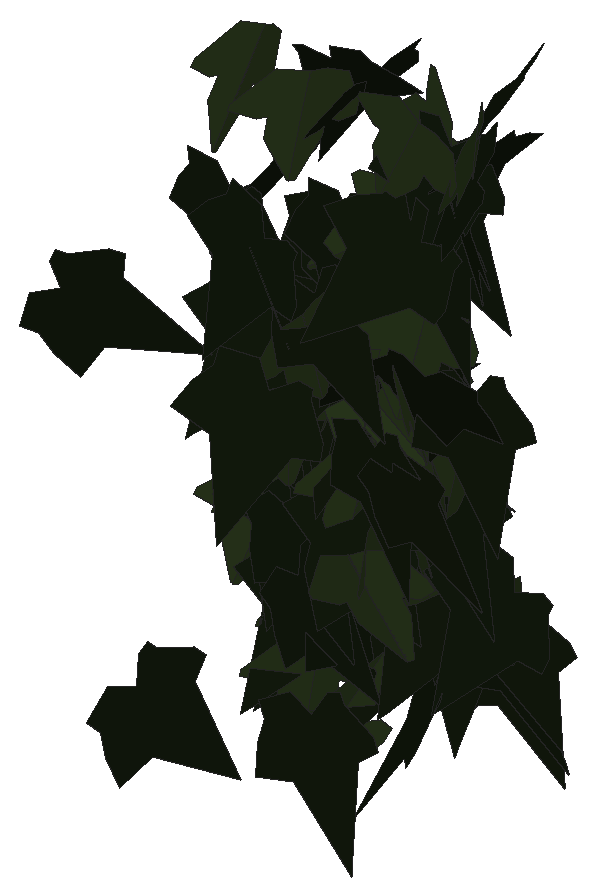
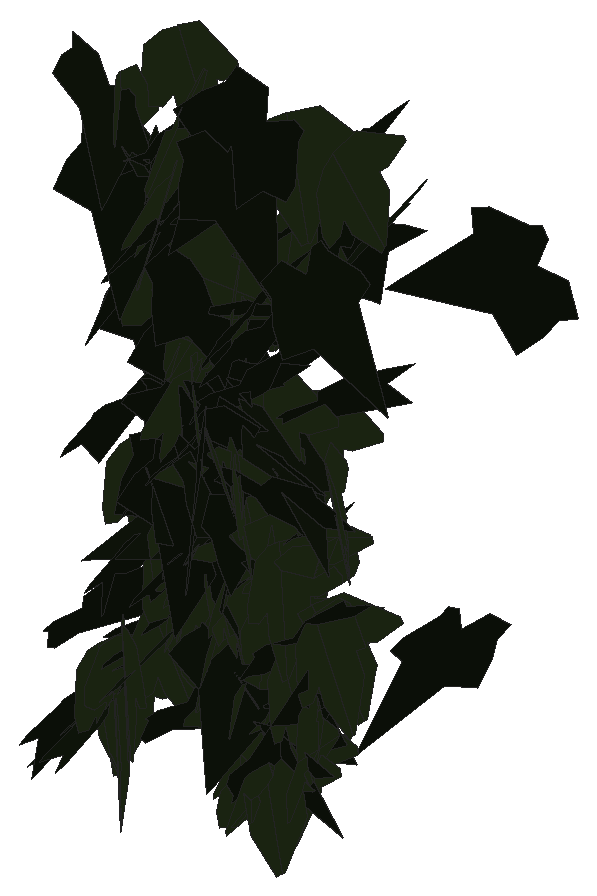
# SketchUp Ruby script. Lengths in inches.
U = 1.inch
M = Sketchup.active_model
def pt(a) = Geom::Point3d.new(a.map { |v| v * U })
def face(e, loops, mat)
  f = e.add_face(loops[0].map { |a| pt(a) })
  loops[1..].each { |l| e.add_face(l.map { |a| pt(a) }).erase! }
  f.material = f.back_material = mat if mat
  f
end
# faces: each face lists its corners as indices into pts; further lists are holes
def faces(e, pts, list, mat = nil) = list.each { |f| face(e, (f[0].is_a?(Array) ? f : [f]).map { |l| l.map { |i| pts[i] } }, mat) }
# xy, xz, yz: faces in a plane at the given z, y or x. An outline is a flat list of corners, or four numbers for a rectangle; further outlines are holes
def ring(l) = l.size == 4 ? [[l[0], l[1]], [l[2], l[1]], [l[2], l[3]], [l[0], l[3]]] : l.each_slice(2).to_a
def flat(e, list, mat, &to3) = list.each { |f| face(e, (f[0].is_a?(Array) ? f : [f]).map { |l| ring(l).map { |u, v| to3.(u, v) } }, mat) }
def xy(e, z, list, mat = nil) = flat(e, list, mat) { |x, y| [x, y, z] }
def xz(e, y, list, mat = nil) = flat(e, list, mat) { |x, z| [x, y, z] }
def yz(e, x, list, mat = nil) = flat(e, list, mat) { |y, z| [x, y, z] }
def lines(e, pts, list) = list.each { |a, b| e.add_line(pt(pts[a]), pt(pts[b])) }
# prism: a flat outline (further loops are holes) pulled along v
def prism(e, loops, v, mat = nil)
  f = face(e, loops, mat); d = Geom::Vector3d.new(v.map { |x| x * U })
  f.pushpull(f.normal.samedirection?(d) ? d.length : -d.length)
end
def box(e, o, s, mat = nil) = prism(e, [[o, [o[0] + s[0], o[1], o[2]], [o[0] + s[0], o[1] + s[1], o[2]], [o[0], o[1] + s[1], o[2]]]], [0, 0, s[2]], mat)
def at(x, y, z, deg = 0) = Geom::Transformation.translation(pt([x, y, z])) * Geom::Transformation.rotation(ORIGIN, Z_AXIS, deg.degrees)
def axes(o, x, y, z) = Geom::Transformation.new([*x, 0, *y, 0, *z, 0, *pt(o).to_a, 1])
def part(name) = M.definitions.add(name)
# library, detail: a bought-in or finely detailed component or shape, given as its bounding box
def library(name, o, s) = part(name).tap { |d| box(d.entities, o, s) }
def detail(e, o, s) = box(e.add_group.entities, o, s)
def put(e, d, t, mat = nil) = e.add_instance(d, t).tap { |i| i.material = mat if mat }
def group(e, t, mat = nil) = e.add_group.tap { |g| g.transformation = t; g.material = mat if mat }.entities
root = M.entities
M.materials.add("efeu1").color = [18, 25, 13]
M.materials.add("efeu2").color = [43, 57, 29]
c1 = part("ivyleaf_10")
p = [[0,0.5,-0.03],[-0.0625,2.02,-0.43],[-0.19,2.01,-0.46],[-0.54,1.05,-0.29],[-0.52,0.625,-0.18],[-0.83,0.76,-0.28],
  [-1.16,0.64,-0.33],[-1.15,0.33,-0.24],[-0.77,-0.39,0.02],[-0.3,-0.51,0.16],[0.04,-0.48,0.23],[-0.02,2.01,-0.4375],
  [-0.06,2.01,-0.43],[0.04,-0.49,0.23],[0.67,-0.49,0.14],[1.38,0.36,-0.2],[1.375,0.51,-0.24],[0.81,0.65,-0.19],
  [0.62,0.59,-0.15],[0.6,1.09,-0.28],[0.5,1.23,-0.31]]
faces(c1.entities,p,[[0,1,2,3,4,5,6,7,8,9,10],[11,12,0,13,14,15,16,17,18,19,20]],"efeu2")
c2 = part("ivyleaf_9")
p = [[1.54,2.16,1.25],[1.36,2.04,1.19],[-0.21,0.99,0.68],[-0.71,1.11,0.82],[-0.85,0.86,0.67],[-0.8,0.17,0.21],
  [-0.9,-0.01,0.1],[-0.67,-0.16,-0.02],[-0.08,-0.08,-0.05],[-0.03,-0.6,-0.4],[0.65,-0.88,-0.66],[0.83,-0.6,-0.49],
  [1.29,-0.42,-0.43],[1.8125,-0.07,-0.26],[1.21,0.44,0.15]]
faces(c2.entities,p,[[0,1,2,3,4,5,6,7,8,9,10,11,12,13,14]],"efeu1")
put(root,c1,axes([19.44,222.39,243.55],[-0.01108,-0.49032,0.09727],[0.0069,-0.09743,-0.49037],[0.49983,-0.00952,0.00893]))
put(root,c2,axes([19.07,219.82,246.48],[0.1213,0.02445,-0.48445],[0.28717,0.39883,0.09203],[0.39092,-0.30056,0.08272]))
put(root,c1,axes([19.42,222.27,245.14],[0.30029,-0.39808,0.03688],[0.05716,-0.0029,-0.49671],[0.39568,0.30253,0.04376]))
put(root,c1,axes([19.6,222.22,243.52],[-0.27833,-0.36558,0.19719],[-0.0556,-0.20243,-0.45379],[0.41163,-0.27454,0.07203]))
put(root,c1,axes([19.41,222.78,242.53],[-0.01774,0.17283,-0.46884],[0.04454,-0.46673,-0.17373],[-0.4977,-0.04793,0.00117]))
put(root,c1,axes([19.51,221.99,248.25],[-0.02394,-0.44074,0.23489],[0.06215,-0.23596,-0.43642],[0.49555,0.0083,0.06608]))
put(root,c2,axes([19.79,222.18,247.12],[-0.2297,0.38883,-0.2146],[0.05063,-0.2171,-0.44755],[-0.44122,-0.22733,0.06036]))
put(root,c1,axes([19.65,222.62,243.16],[0.06523,-0.49538,0.01862],[-0.00038,-0.01883,-0.49965],[0.49573,0.06517,-0.00284]))
put(root,c2,axes([19.8,222.8,242.26],[-0.17445,-0.39074,0.25862],[0.10442,0.23661,0.42792],[-0.4568,0.20331,-0.00095]))
put(root,c1,axes([19.82,222.78,242.22],[-0.21532,-0.44772,0.05641],[-0.00416,-0.06054,-0.4963],[0.45124,-0.21419,0.02235]))
put(root,c2,axes([19.69,222.5,243.53],[-0.13385,-0.48058,0.03356],[-0.00506,-0.03343,-0.49886],[0.48172,-0.13388,0.00408]))
put(root,c1,axes([19.87,222.46,244.17],[-0.04913,-0.4925,-0.07091],[0.00897,0.07037,-0.49494],[0.4975,-0.04991,0.00192]))
put(root,c1,axes([19.83,222.76,242.27],[-0.0214,0.43846,-0.23937],[-0.0254,-0.24024,-0.43777],[-0.4989,-0.00657,0.03255]))
put(root,c2,axes([20.02,222.71,242.46],[-0.48575,-0.09263,-0.07392],[0.07164,0.01896,-0.49448],[0.09441,-0.49098,-0.00515]))
put(root,c1,axes([19.79,222.09,244.13],[0.15451,0.47129,0.06333],[0.02774,0.05754,-0.4959],[-0.47472,0.15676,-0.00836]))
put(root,c2,axes([19.79,220.01,242.45],[0.12581,-0.20795,-0.43696],[-0.10901,0.4277,-0.23493],[0.47148,0.15437,0.06228]))
put(root,c1,axes([20.26,222.06,244.17],[0.15449,0.07499,0.46958],[-0.43453,-0.17831,0.17143],[0.19317,-0.46107,0.01008]))
put(root,c1,axes([20,222.74,242.77],[0.04949,-0.47561,-0.14609],[0.00177,0.14698,-0.47791],[0.49754,0.04679,0.01623]))
put(root,c2,axes([20.02,222.51,242.54],[-0.29711,-0.387,0.10934],[-0.07569,-0.0797,-0.48777],[0.39496,-0.3064,-0.01122]))
put(root,c2,axes([19.98,221.75,245.61],[-0.27657,-0.37553,0.18025],[-0.03623,-0.19385,-0.45947],[0.41497,-0.2672,0.08002]))
put(root,c1,axes([19.91,222.74,242.55],[-0.02184,0.47886,-0.14219],[-0.00742,-0.14262,-0.47917],[-0.49947,-0.01882,0.01334]))
put(root,c2,axes([20.31,221.9,245.15],[-0.17916,0.44858,0.12916],[-0.09313,0.10122,-0.48071],[-0.45742,-0.1963,0.04729]))
put(root,c2,axes([20.17,222.72,243.14],[0.04789,0.44383,0.22522],[-0.01794,0.22765,-0.44481],[-0.49738,0.03452,0.03773]))
put(root,c2,axes([19.82,221.3125,247.09],[0.05028,-0.46421,0.17883],[0.06656,-0.17185,-0.4648],[0.49299,0.07054,0.04452]))
put(root,c2,axes([20.06,222.5,244.98],[-0.37971,-0.25936,-0.19636],[0.1894,0.06913,-0.45755],[0.26448,-0.42185,0.04575]))
put(root,c1,axes([20.14,222.54,242.63],[-0.07016,-0.46182,-0.17832],[0.02959,0.17586,-0.46711],[0.49417,-0.07609,0.00265]))
put(root,c1,axes([20.23,222.07,242.07],[-0.29212,-0.40137,0.05969],[-0.02394,-0.05638,-0.49623],[0.40508,-0.29278,0.01372]))
put(root,c1,axes([20.09,222.56,242.85],[0.239,0.43915,0.00562],[-0.01394,0.01398,-0.49961],[-0.43896,0.23865,0.01892]))
put(root,c1,axes([20.28,222.78,243.11],[0.11009,-0.48542,0.04737],[0.00036,-0.04848,-0.49764],[0.48773,0.10961,-0.01032]))
put(root,c1,axes([20.33,222.53,243.49],[-0.24429,-0.43621,0.0064],[0.00558,-0.01046,-0.49986],[0.43622,-0.24415,0.00998]))
put(root,c1,axes([20.26,222.62,244.34],[0.29357,0.36079,-0.18344],[-0.11088,-0.14625,-0.4651],[-0.38926,0.31375,-0.00587]))
put(root,c1,axes([20.35,221.75,248.21],[-0.28011,-0.4076,0.07346],[-0.01306,-0.07995,-0.49339],[0.41396,-0.27833,0.03414]))
put(root,c1,axes([20.32,222.48,244.96],[0.18695,-0.45958,-0.06195],[0.00746,0.06976,-0.49505],[0.46368,0.18417,0.03294]))
put(root,c1,axes([20.33,222.66,243.72],[0.0864,-0.36412,-0.33159],[0.03489,0.34033,-0.36463],[0.49124,0.03987,0.08422]))
put(root,c2,axes([20.41,222.58,244.78],[-0.27135,0.21259,-0.36218],[0.24815,-0.26671,-0.34247],[-0.33881,-0.36561,0.03923]))
put(root,c1,axes([20.41,221.39,245.09],[-0.23966,-0.4372,-0.03767],[0.01803,0.03308,-0.49858],[0.43845,-0.24033,-0.00009]))
put(root,c1,axes([20.31,222.57,244.125],[-0.32616,-0.29253,-0.24092],[0.18513,0.15436,-0.43806],[0.33067,-0.37496,0.00762]))
put(root,c1,axes([20.67,222.54,244.81],[-0.34121,-0.12798,0.34234],[-0.29268,-0.1848,-0.36081],[0.21889,-0.44662,0.0512]))
put(root,c2,axes([20.26,222.43,243.96],[-0.03911,-0.4848,0.11593],[0.01186,-0.11716,-0.48594],[0.49833,-0.03526,0.02066]))
put(root,c1,axes([20.53,221.96,245.49],[-0.40967,-0.27833,0.06855],[-0.05406,-0.0424,-0.49526],[0.28151,-0.4132,0.00465]))
put(root,c2,axes([20.24,222.33,246.53],[0.09876,-0.48312,-0.08273],[-0.02283,0.07976,-0.49307],[0.48962,0.10116,-0.0063]))
put(root,c1,axes([20.45,222.65,243.97],[0.15813,-0.46926,0.06925],[0.01817,-0.06695,-0.49516],[0.47399,0.15911,-0.00412]))
put(root,c2,axes([20.41,222.28,243.5625],[-0.17795,-0.42442,0.19545],[-0.03274,-0.1973,-0.45826],[0.46611,-0.1759,0.04243]))
put(root,c2,axes([20.65,222.28,248.15],[-0.13614,0.4645,-0.12533],[0.01024,-0.12742,-0.48338],[-0.481,-0.13418,0.02518]))
put(root,c2,axes([20.72,222.42,244.83],[-0.29607,0.39524,-0.07831],[0.01755,-0.08444,-0.49251],[-0.40254,-0.29438,0.03612]))
put(root,c2,axes([20.45,222.34,245.87],[-0.16839,-0.46104,0.09532],[-0.00206,-0.10051,-0.48979],[0.47079,-0.16535,0.03195]))
put(root,c1,axes([20.53,222.7,242.94],[0.47155,-0.15182,-0.06775],[-0.06398,0.02235,-0.49539],[0.15345,0.47587,0.00165]))
put(root,c1,axes([20.58,221.81,243.1875],[-0.01597,-0.49709,-0.05147],[0.00979,0.05118,-0.49728],[0.49965,-0.01689,0.00809]))
put(root,c2,axes([20.38,221.53,243.8125],[0.18912,-0.43981,-0.14423],[-0.02541,0.1457,-0.47763],[0.46216,0.18799,0.03275]))
put(root,c2,axes([20.56,222.25,245.15],[-0.37621,-0.24187,-0.22352],[0.25262,0.00578,-0.43145],[0.21129,-0.43757,0.11786]))
put(root,c2,axes([20.49,222.02,248.4375],[0.47303,0.15077,-0.05925],[-0.06593,0.01214,-0.49549],[-0.14797,0.47657,0.03136]))
put(root,c2,axes([20.47,222.23,246.58],[0.03775,-0.47721,0.14437],[-0.00067,-0.14483,-0.47856],[0.49857,0.03594,-0.01158]))
put(root,c2,axes([20.73,222.54,244.79],[0.12815,0.48264,0.02521],[-0.00525,0.02747,-0.49922],[-0.48327,0.12768,0.01211]))
put(root,c1,axes([20.53,222,244.99],[-0.40635,-0.15797,-0.24479],[0.23483,0.07106,-0.43567],[0.17243,-0.46904,0.01644]))
put(root,c1,axes([20.65,222.48,245.18],[0.31296,-0.38967,0.01466],[0.00471,-0.01502,-0.49975],[0.38991,0.31295,-0.00573]))
put(root,c1,axes([20.59,222.34,245.07],[0.33798,-0.36769,-0.0239],[0.08857,0.11255,-0.47905],[0.35767,0.31958,0.14122]))
put(root,c2,axes([20.83,222.5625,245.08],[0.21202,0.33327,-0.30656],[-0.21063,-0.22707,-0.39253],[-0.40085,0.29559,0.04411]))
put(root,c2,axes([20.79,222.33,245.73],[-0.35685,-0.32402,0.13293],[-0.06809,-0.12197,-0.48009],[0.34354,-0.36075,0.04292]))
put(root,c1,axes([20.67,222.31,243.91],[-0.19108,-0.42513,-0.18098],[0.12484,0.14106,-0.46316],[0.44487,-0.22218,0.05224]))
put(root,c2,axes([20.85,222.4,245.19],[0.14781,-0.07938,-0.47101],[-0.43443,0.18261,-0.16711],[0.19855,0.45864,-0.01499]))
put(root,c1,axes([20.65,222.61,244.23],[-0.09798,0.48155,-0.09224],[0.02822,-0.08837,-0.49132],[-0.48949,-0.10148,-0.00987]))
put(root,c2,axes([20.49,220.87,246.72],[0.08299,-0.19606,0.45241],[0.16082,-0.42292,-0.21278],[0.4661,0.18083,-0.00714]))
put(root,c2,axes([20.98,222.48,244.66],[-0.2317,0.43701,-0.0731],[0.04618,-0.05822,-0.49445],[-0.44066,-0.23587,-0.01338]))
put(root,c2,axes([20.64,221.93,242.79],[-0.08495,-0.2996,0.39118],[0.0647,-0.4003,-0.29254],[0.48846,0.00091,0.10678]))
put(root,c1,axes([20.83,222.01,244.32],[-0.13573,-0.46731,0.1149],[0.02859,-0.12701,-0.48275],[0.48038,-0.12448,0.0612]))
put(root,c2,axes([20.75,220.58,247.26],[-0.0847,-0.41999,0.25775],[-0.05127,-0.25259,-0.42845],[0.4901,-0.09901,-0.00027]))
put(root,c1,axes([21.08,222.36,246.82],[-0.11343,-0.17,0.45632],[-0.25151,-0.38076,-0.20437],[0.41698,-0.27591,0.00086]))
put(root,c2,axes([20.8,222.66,242.55],[-0.19954,-0.44635,0.10465],[-0.01141,-0.10926,-0.48778],[0.45832,-0.19705,0.03341]))
put(root,c1,axes([20.76,222.56,244.73],[0.2168,0.38763,0.22966],[0.00996,0.25068,-0.43251],[-0.45044,0.19211,0.10097]))
put(root,c2,axes([20.9,222.22,246.38],[-0.35759,-0.3463,0.04694],[0.0389,-0.10618,-0.48704],[0.34729,-0.34468,0.10288]))
put(root,c2,axes([20.72,221.23,243.38],[0.25285,-0.33028,-0.27746],[-0.12544,0.25141,-0.41359],[0.41271,0.27876,0.04428]))
put(root,c2,axes([20.68,222.79,244.24],[0.11433,-0.48223,-0.06621],[0.00902,0.0701,-0.49498],[0.48667,0.11199,0.02473]))
put(root,c2,axes([20.94,222.05,243.6875],[-0.28575,-0.38621,0.13852],[-0.07885,-0.11396,-0.48041],[0.40265,-0.2964,0.00423]))
put(root,c1,axes([20.8125,221.46,241.59],[-0.08473,-0.42835,0.24359],[0.04011,0.24035,0.4366],[-0.49113,0.09352,-0.00637]))
put(root,c1,axes([21.01,222.42,243.86],[-0.2823,-0.36867,0.18544],[-0.06568,-0.18168,-0.46117],[0.40742,-0.28474,0.05415]))
put(root,c2,axes([21.0625,222.31,246.89],[-0.17276,0.3963,-0.2512],[0.11427,-0.22409,-0.43212],[-0.45508,-0.20672,-0.01314]))
put(root,c2,axes([21.09,222.41,245.55],[-0.47771,-0.13089,-0.06829],[0.06547,0.0195,-0.49531],[0.13232,-0.48217,-0.00149]))
put(root,c1,axes([20.99,222.3,245.66],[0.21326,-0.44513,-0.07985],[0.01109,0.0934,-0.49107],[0.4521,0.20768,0.04971]))
put(root,c2,axes([20.82,222.54,245.51],[-0.22081,-0.22187,-0.38989],[0.279,0.27238,-0.313],[0.35129,-0.35579,0.00351]))
put(root,c2,axes([20.6875,222.59,244.59],[0.431,-0.24877,0.04846],[0.10378,0.086,-0.48149],[0.23123,0.42511,0.12577]))
put(root,c1,axes([21.03,222.46,245.65],[-0.09934,0.48517,0.06889],[-0.07529,0.05435,-0.4913],[-0.48421,-0.10798,0.06226]))
put(root,c1,axes([21,221.83,246.83],[-0.35166,0.32937,-0.13361],[0.04985,-0.14039,-0.47729],[-0.35193,-0.34901,0.0659]))
put(root,c1,axes([21.04,222.04,246.42],[-0.46367,0.08486,-0.16677],[0.1659,-0.01963,-0.47126],[-0.08654,-0.49235,-0.00995]))
put(root,c1,axes([21.15,220.72,246.43],[-0.09944,-0.45925,-0.1709],[0.05084,0.16377,-0.46967],[0.48737,-0.11078,0.01412]))
put(root,c1,axes([21.13,222.32,243.65],[-0.32561,0.3674,-0.09484],[0.05905,-0.07438,-0.4909],[-0.37482,-0.33088,0.00505]))
put(root,c1,axes([20.82,221.87,245.23],[0.22743,0.04939,0.44253],[0.43576,0.07751,-0.23261],[-0.09158,0.49148,-0.00779]))
put(root,c2,axes([21.01,222.59,245.01],[0.10976,-0.48774,-0.00756],[-0.00753,0.00605,-0.49991],[0.48775,0.10986,-0.00601]))
put(root,c1,axes([21.49,222.14,244.6],[-0.24431,0.16957,0.40194],[-0.36625,0.17055,-0.29457],[-0.237,-0.43836,0.04088]))
put(root,c2,axes([21.33,221.62,245.74],[0.13573,0.48035,-0.02898],[-0.00889,-0.0276,-0.49916],[-0.48114,0.13602,0.00105]))
put(root,c2,axes([21.23,220.0625,246.03],[-0.22668,-0.44566,0.00276],[-0.00241,-0.00186,-0.49999],[0.44566,-0.22669,-0.0013]))
put(root,c1,axes([21.33,221.56,244.08],[0.20483,-0.41152,-0.19671],[0.02003,0.22354,-0.4468],[0.45568,0.17515,0.10806]))
put(root,c2,axes([21.09,222.71,243.1],[0.32576,-0.32061,-0.20271],[-0.04363,0.23376,-0.43983],[0.37679,0.30425,0.12432]))
put(root,c2,axes([21.11,220.96,246.61],[0.18673,-0.43657,-0.15665],[0.00245,0.1698,-0.47028],[0.46382,0.17486,0.06555]))
put(root,c1,axes([21.36,222.99,242.31],[0.23296,-0.41817,-0.14443],[-0.0003,0.16308,-0.47266],[0.44242,0.2203,0.07573]))
put(root,c1,axes([21.41,222.3125,242.9375],[-0.0176,-0.48078,0.13615],[-0.00201,-0.13617,-0.4811],[0.49969,-0.01748,0.00286]))
put(root,c1,axes([21.37,222.86,242.96],[0.34498,-0.3501,-0.09175],[0.01418,0.13973,-0.47987],[0.36165,0.32848,0.10634]))
put(root,c1,axes([21.41,222.3,247.75],[-0.153,0.34519,0.32777],[0.13808,-0.2973,0.37755],[0.45555,0.20604,-0.00435]))
put(root,c1,axes([21.45,222.29,247.48],[-0.15441,0.47462,0.02996],[-0.0112,0.02786,-0.4991],[-0.47543,-0.1548,0.00203]))
put(root,c1,axes([21.44,221.22,243.73],[-0.46008,-0.10652,-0.16426],[0.16125,0.03172,-0.47222],[0.11102,-0.48749,0.00517]))
put(root,c1,axes([21.5625,222.61,242.66],[-0.12105,-0.46542,-0.13686],[0.02198,0.13565,-0.48074],[0.48463,-0.12241,-0.01238]))
put(root,c2,axes([21.52,222.37,243.06],[-0.21199,-0.42707,0.15057],[-0.02538,-0.15478,-0.47476],[0.45212,-0.20894,0.04395]))
put(root,c1,axes([21.62,222.88,242.68],[-0.02173,-0.49923,0.0173],[0.00001,-0.01732,-0.4997],[0.49953,-0.02171,0.00076]))
put(root,c1,axes([21.59,221.64,245.76],[-0.22429,0.44196,0.0661],[-0.04003,0.05379,-0.49548],[-0.44507,-0.22756,0.01125]))
put(root,c2,axes([21.45,222.33,247.14],[0.21478,-0.35952,-0.27316],[-0.11961,0.24638,-0.41832],[0.43539,0.24504,0.01984]))
put(root,c2,axes([21.43,222.53,244.03],[0.1413,-0.46343,-0.12356],[-0.03482,0.11856,-0.48449],[0.47835,0.14552,0.00123]))
put(root,c1,axes([21.68,222.31,244.59],[-0.08001,-0.49283,0.02678],[-0.00335,-0.02659,-0.49928],[0.49355,-0.08007,0.00096]))
put(root,c1,axes([21.91,221.4,248.42],[-0.42469,-0.01551,0.26343],[-0.26044,-0.05574,-0.42316],[0.04249,-0.49664,0.03927]))
put(root,c2,axes([21.48,220.44,242.52],[0.09365,-0.47916,-0.10787],[0.00146,0.11009,-0.48773],[0.49115,0.09104,0.02202]))
put(root,c1,axes([21.82,221.62,246.25],[-0.36543,-0.31934,0.12036],[-0.06234,-0.11091,-0.48354],[0.33552,-0.36841,0.04124]))
put(root,c2,axes([21.55,222.52,242.84],[0.01317,-0.49584,0.06302],[-0.00321,-0.06312,-0.49599],[0.49982,0.01266,-0.00484]))
put(root,c2,axes([21.84,222.24,247.63],[0.03306,0.4977,0.03471],[0.00024,0.03477,-0.49879],[-0.49891,0.033,0.00206]))
put(root,c2,axes([21.92,221.625,242.39],[-0.38329,0.24794,-0.204],[0.16332,-0.12295,-0.4563],[-0.27643,-0.41643,0.01326]))
put(root,c2,axes([21.68,222.2,247.8125],[-0.07015,-0.49189,0.05584],[-0.01123,-0.05481,-0.49686],[0.49493,-0.07097,-0.00336]))
put(root,c2,axes([21.93,221.39,247.29],[-0.3717,-0.28252,0.17895],[-0.06461,-0.20184,-0.45287],[0.32812,-0.35978,0.11354]))
put(root,c2,axes([21.63,221.98,247.05],[0.17372,-0.46835,-0.02162],[-0.00947,0.01955,-0.49953],[0.46876,0.17396,-0.00208]))
put(root,c2,axes([21.58,222.93,242.36],[0.30917,-0.3922,-0.02424],[0.02299,0.04885,-0.49708],[0.39228,0.30625,0.04824]))
put(root,c2,axes([21.65,221.15,245.09],[0.16773,-0.46831,0.05052],[0.01419,-0.04858,-0.49743],[0.47081,0.1683,-0.003]))
put(root,c2,axes([22.15,222.19,248.31],[-0.05415,0.421,0.26425],[-0.05376,0.25929,-0.42412],[-0.49414,-0.07434,0.01718]))
put(root,c2,axes([22.07,221.36,245.92],[0.32646,0.21315,-0.31304],[-0.28718,-0.1301,-0.38808],[-0.24689,0.43318,0.03748]))
put(root,c2,axes([22.22,221.87,247.8125],[-0.40719,0.28575,-0.05048],[0.03843,-0.0331,-0.49742],[-0.28761,-0.40897,0.00499]))
put(root,c2,axes([21.79,222.9375,242.4],[0.12577,-0.4515,-0.17415],[-0.00678,0.17828,-0.46709],[0.48388,0.11985,0.03872]))
put(root,c2,axes([21.7,222.26,247.28],[0.19241,-0.04184,-0.4596],[0.44129,-0.12904,0.19649],[-0.13505,-0.48125,-0.01273]))
put(root,c2,axes([21.87,222.32,245.2],[0.07127,-0.49182,-0.05506],[-0.00551,0.05483,-0.49695],[0.49486,0.07144,0.0024]))
put(root,c2,axes([22.05,222.625,243.09],[-0.20003,-0.41063,0.2034],[-0.06069,-0.19624,-0.45586],[0.45421,-0.20706,0.02867]))
put(root,c2,axes([21.82,221.24,244.84],[0.32668,-0.35486,-0.13173],[-0.0415,0.13938,-0.47838],[0.37624,0.32349,0.06161]))
put(root,c1,axes([22.1,221.99,248.13],[0.15585,-0.46108,-0.11452],[0.01199,0.12431,-0.48415],[0.47494,0.14817,0.04981]))
